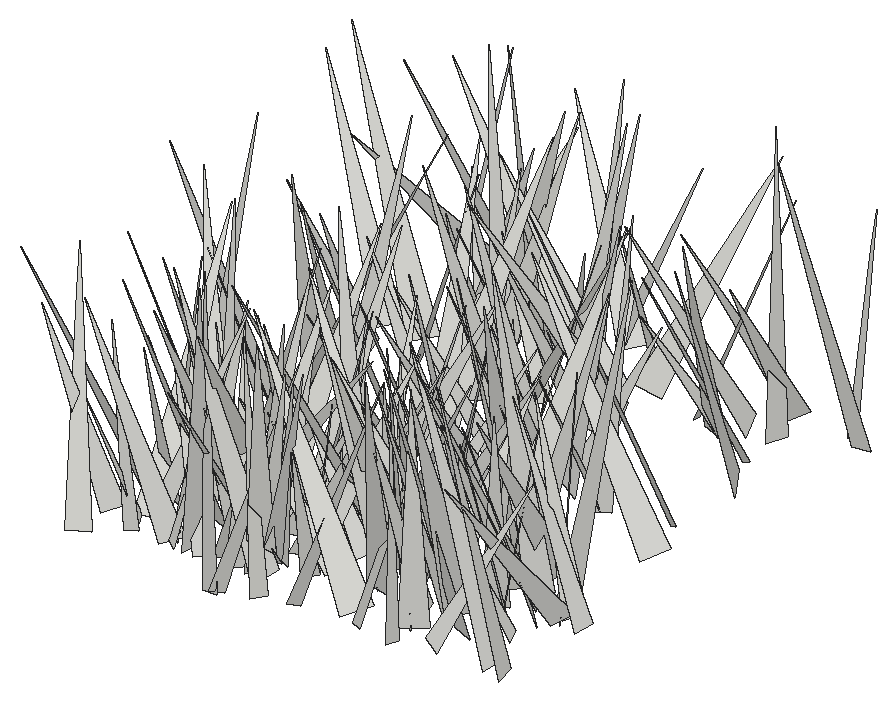
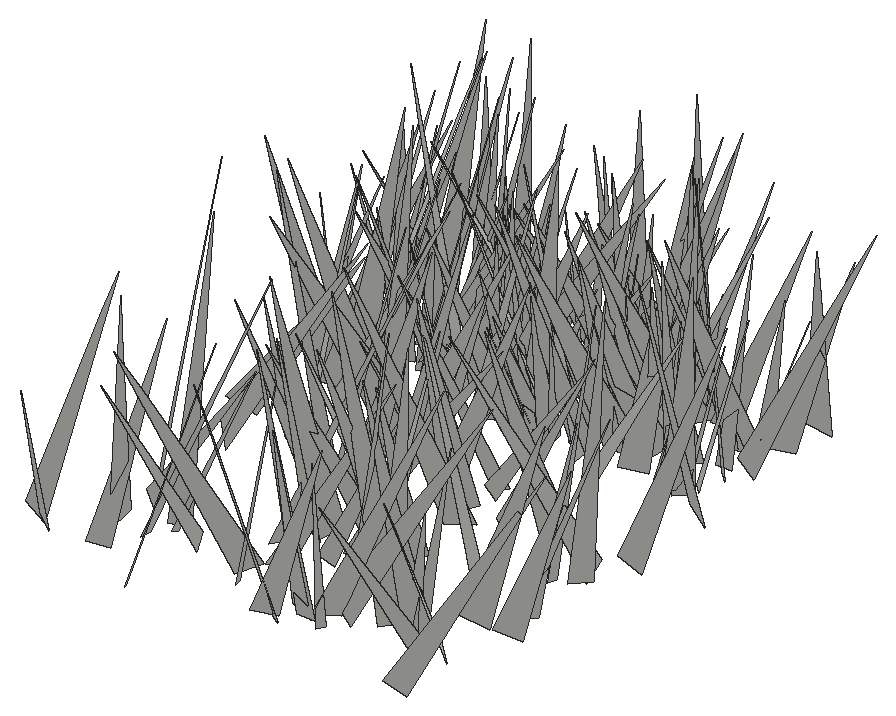
# SketchUp Ruby script. Lengths in inches.
U = 1.inch
M = Sketchup.active_model
def pt(a) = Geom::Point3d.new(a.map { |v| v * U })
def face(e, loops, mat)
  f = e.add_face(loops[0].map { |a| pt(a) })
  loops[1..].each { |l| e.add_face(l.map { |a| pt(a) }).erase! }
  f.material = f.back_material = mat if mat
  f
end
# faces: each face lists its corners as indices into pts; further lists are holes
def faces(e, pts, list, mat = nil) = list.each { |f| face(e, (f[0].is_a?(Array) ? f : [f]).map { |l| l.map { |i| pts[i] } }, mat) }
# xy, xz, yz: faces in a plane at the given z, y or x. An outline is a flat list of corners, or four numbers for a rectangle; further outlines are holes
def ring(l) = l.size == 4 ? [[l[0], l[1]], [l[2], l[1]], [l[2], l[3]], [l[0], l[3]]] : l.each_slice(2).to_a
def flat(e, list, mat, &to3) = list.each { |f| face(e, (f[0].is_a?(Array) ? f : [f]).map { |l| ring(l).map { |u, v| to3.(u, v) } }, mat) }
def xy(e, z, list, mat = nil) = flat(e, list, mat) { |x, y| [x, y, z] }
def xz(e, y, list, mat = nil) = flat(e, list, mat) { |x, z| [x, y, z] }
def yz(e, x, list, mat = nil) = flat(e, list, mat) { |y, z| [x, y, z] }
def lines(e, pts, list) = list.each { |a, b| e.add_line(pt(pts[a]), pt(pts[b])) }
# prism: a flat outline (further loops are holes) pulled along v
def prism(e, loops, v, mat = nil)
  f = face(e, loops, mat); d = Geom::Vector3d.new(v.map { |x| x * U })
  f.pushpull(f.normal.samedirection?(d) ? d.length : -d.length)
end
def box(e, o, s, mat = nil) = prism(e, [[o, [o[0] + s[0], o[1], o[2]], [o[0] + s[0], o[1] + s[1], o[2]], [o[0], o[1] + s[1], o[2]]]], [0, 0, s[2]], mat)
def at(x, y, z, deg = 0) = Geom::Transformation.translation(pt([x, y, z])) * Geom::Transformation.rotation(ORIGIN, Z_AXIS, deg.degrees)
def axes(o, x, y, z) = Geom::Transformation.new([*x, 0, *y, 0, *z, 0, *pt(o).to_a, 1])
def part(name) = M.definitions.add(name)
# library, detail: a bought-in or finely detailed component or shape, given as its bounding box
def library(name, o, s) = part(name).tap { |d| box(d.entities, o, s) }
def detail(e, o, s) = box(e.add_group.entities, o, s)
def put(e, d, t, mat = nil) = e.add_instance(d, t).tap { |i| i.material = mat if mat }
def group(e, t, mat = nil) = e.add_group.tap { |g| g.transformation = t; g.material = mat if mat }.entities
root = M.entities
c1 = part("fur_instance\#9")
p = [[0.8125,0,1.79],[0.67,-0.02,1.48],[0,-0.11,0],[0,0.11,0]]
faces(c1.entities,p,[[0,1,2,3]])
put(root,c1,axes([460.6875,140.12,-21.86],[7.59105,-2.36712,2.02897],[-2.18853,-7.84946,-0.96967],[-2.22043,-0.35586,7.89221]))
put(root,c1,axes([464.49,140.16,-21.86],[5.8288,-3.89293,1.62458],[-3.86791,-6.0381,-0.59132],[-1.68328,0.3943,6.98428]))
put(root,c1,axes([463.9375,137.01,-21.86],[2.76553,6.92914,2.18566],[6.51494,-3.40021,2.53621],[-3.21647,-0.92942,7.01632]))
put(root,c1,axes([464.78,140.87,-21.66],[-1.76635,-5.02439,0.02248],[-4.81779,1.68692,-1.51928],[-1.42615,0.52421,5.10454]))
put(root,c1,axes([455.63,140.11,-21.66],[-4.26864,3.3889,1.68719],[3.78174,3.93314,1.66776],[0.17248,-2.36607,5.18889]))
put(root,c1,axes([459.45,139.79,-21.86],[-3.27496,5.22829,1.96451],[5.47571,2.5569,2.32348],[-1.10043,-2.83671,5.71505]))
put(root,c1,axes([462.74,142,-21.86],[0.98136,-7.62341,0.77855],[-7.49654,-1.11781,-1.49599],[-1.58884,0.56543,7.53933]))
put(root,c1,axes([470.25,142.0625,-21.86],[0.34985,-8.1007,0.677],[-7.9597,-0.20383,1.67442],[1.6501,0.73429,7.93347]))
put(root,c1,axes([465.12,139.72,-21.86],[-8.06314,0.9505,0.88883],[1.02226,8.07835,0.63476],[0.80526,-0.7379,8.09412]))
put(root,c1,axes([479.77,139.47,-21.86],[-7.02647,-2.17808,1.10616],[-2.29777,7.03636,-0.74079],[0.82938,1.04138,7.31892]))
put(root,c1,axes([456.98,140.48,-21.86],[-3.14416,-1.79317,0.28571],[-1.75542,3.14785,0.43854],[0.46429,-0.24163,3.59289]))
put(root,c1,axes([455.63,137.48,-21.66],[-1.06159,6.87885,0.56166],[6.76624,0.92524,1.45707],[-1.36093,-0.76575,6.80607]))
put(root,c1,axes([474.82,142.48,-21.66],[5.51708,-5.76072,0.82028],[-5.55442,-5.55067,-1.6234],[-1.73412,-0.54876,7.80952]))
put(root,c1,axes([464.41,136.92,-21.66],[5.42,0.95377,1.93695],[-0.10115,-5.11614,2.80228],[-2.15667,2.63692,4.73638]))
put(root,c1,axes([473.36,141.42,-21.66],[-6.08575,-1.31512,1.93305],[-0.80976,6.24223,1.69745],[2.19329,-1.34444,5.99037]))
put(root,c1,axes([473.63,140.26,-21.86],[4.24659,-4.94069,2.32668],[-5.22174,-4.53655,-0.10277],[-1.59916,1.69313,6.51409]))
put(root,c1,axes([466.03,138.0625,-21.86],[-6.21207,0.31771,0.7174],[0.09871,5.99609,-1.80072],[0.77837,1.77522,5.95384]))
put(root,c1,axes([473.68,138.58,-21.86],[-5.20455,-0.25594,1.25726],[-0.61037,5.11409,-1.48563],[1.12857,1.58561,4.99457]))
put(root,c1,axes([475.7,141.32,-21.86],[-3.27464,-6.78559,1.40651],[-6.92909,3.22889,-0.5548],[0.10135,1.50857,7.51397]))
put(root,c1,axes([466.7,141.1,-21.86],[2.8154,-3.04723,0.70248],[-2.99803,-2.89898,-0.55973],[-0.88933,0.126,4.11081]))
put(root,c1,axes([478.75,139.99,-21.86],[-8.26176,0.40654,0.83522],[0.41692,8.30295,0.08258],[0.83009,-0.12394,8.27135]))
put(root,c1,axes([464.52,140.88,-21.86],[6.13982,-1.63324,0.91897],[-1.58888,-6.20592,-0.4139],[-0.99371,-0.16841,6.33984]))
put(root,c1,axes([470.73,139.58,-21.66],[-4.85114,5.94494,0.47809],[5.69058,4.42924,2.66526],[-1.78556,-2.03568,7.19529]))
put(root,c1,axes([459.375,140.12,-21.86],[2.36922,2.94645,1.17355],[3.15581,-2.33594,-0.5062],[-0.31572,-1.23846,3.7468]))
put(root,c1,axes([459.64,139.46,-21.86],[2.29816,3.3477,0.63042],[3.39972,-2.30202,-0.16916],[-0.21536,-0.61617,4.05709]))
put(root,c1,axes([464.46,141.57,-21.86],[-0.76172,-5.93829,1.58025],[-5.83151,1.20063,1.7008],[1.93753,1.27903,5.74028]))
put(root,c1,axes([464.05,140.9375,-21.86],[0.25447,-5.59234,1.88155],[-5.79418,0.11887,1.13692],[1.11444,1.89496,5.48146]))
put(root,c1,axes([464.12,141,-21.66],[1.30343,6.50873,4.51627],[7.0846,-3.00591,2.28737],[-3.54523,-3.61388,6.23141]))
put(root,c1,axes([457.35,139.32,-21.86],[0.45308,4.94253,1.25959],[4.74966,-0.86975,1.70432],[-1.859,-1.01755,4.66145]))
put(root,c1,axes([473.06,140.45,-21.86],[3.81307,5.29138,3.34018],[5.75803,-4.49829,0.55278],[-2.44962,-2.33704,6.49867]))
put(root,c1,axes([460.32,142.4,-21.86],[-3.1759,-6.57357,0.78945],[-6.61199,3.10387,-0.75436],[-0.34161,1.03711,7.26148]))
put(root,c1,axes([461.49,139.54,-21.86],[-1.35626,4.67986,0.4324],[4.48876,1.15652,1.56235],[-1.3925,-0.82998,4.61514]))
put(root,c1,axes([474.27,142.13,-21.86],[-5.80555,-2.80529,1.19859],[-2.69051,5.92298,0.83076],[1.43785,-0.24369,6.39405]))
put(root,c1,axes([475.28,139.49,-21.86],[2.06268,4.77096,0.10661],[4.57909,-1.94603,-1.50762],[1.34363,-0.69206,4.97431]))
put(root,c1,axes([455.95,142.52,-21.66],[-2.71774,-6.73125,0.47193],[-6.54696,2.5072,-1.9416],[-1.63394,1.15011,6.99472]))
put(root,c1,axes([464.32,141.84,-21.86],[-3.33376,-1.76985,1.3611],[-1.54667,3.5947,0.88593],[1.61021,-0.21143,3.66899]))
put(root,c1,axes([468.02,138.23,-21.66],[5.42222,1.22065,1.50489],[0.3801,-5.05507,2.73075],[-1.90005,2.47215,4.84081]))
put(root,c1,axes([463.65,139.87,-21.86],[0.20171,6.63601,2.13173],[6.14884,-1.17367,3.07178],[-3.28217,-1.79094,5.8857]))
put(root,c1,axes([457.02,142.83,-21.86],[-0.80762,-5.18,0.70533],[-5.16495,0.90095,0.70267],[0.80822,0.5814,5.19528]))
put(root,c1,axes([477.77,142.53,-21.86],[-4.15133,-1.53142,0.10873],[-1.49707,4.10736,0.69206],[0.34034,-0.61232,4.37033]))
put(root,c1,axes([466.35,141.6,-21.86],[3.95435,2.54343,1.52337],[2.80761,-4.0284,-0.56212],[-0.95239,-1.31514,4.66797]))
put(root,c1,axes([460.26,145.63,-21.86],[7.18044,-3.7228,0.21814],[-3.29243,-6.55088,-3.42221],[-1.75122,-2.94828,7.32847]))
put(root,c1,axes([467.46,142.03,-21.66],[-3.75948,2.94392,0.27379],[2.73653,3.29698,2.12525],[-1.1194,-1.82718,4.27594]))
put(root,c1,axes([461.97,141.26,-21.66],[0.15011,3.96157,1.30257],[3.86973,0.35348,-1.52101],[1.55431,-1.26265,3.66102]))
put(root,c1,axes([478.59,145.29,-21.86],[3.78174,-4.82109,0.17581],[-4.12071,-3.34423,-3.06777],[-2.50869,-1.77444,5.30408]))
put(root,c1,axes([474.12,144.14,-21.66],[-5.52668,-3.91053,1.22579],[-3.5737,5.60606,1.77193],[2.00587,-0.78663,6.53427]))
put(root,c1,axes([463.19,141.96,-21.86],[5.93404,-1.49093,1.99542],[-1.59561,-6.23409,0.08712],[-1.91274,0.57506,6.11785]))
put(root,c1,axes([470.54,144.52,-21.66],[0.16634,-6.6201,0.01552],[-6.42128,-0.15757,1.61124],[1.61035,0.05552,6.42319]))
put(root,c1,axes([474.13,143.64,-21.66],[-7.00038,0.48524,0.02911],[0.47648,6.76613,1.79834],[-0.09628,-1.796,6.78283]))
put(root,c1,axes([477.43,144.62,-21.86],[-4.26482,-5.03014,0.77761],[-4.82923,4.31941,1.45497],[1.60794,-0.36894,6.43227]))
put(root,c1,axes([457.48,141.1,-21.86],[2.30365,5.6713,0.71156],[5.64313,-2.13475,-1.25489],[0.90837,-1.12069,5.9913]))
put(root,c1,axes([475.93,144.27,-21.86],[-3.75985,-4.2409,1.14983],[-3.97997,3.92819,1.47409],[1.86202,-0.16705,5.47255]))
put(root,c1,axes([474.09,143.25,-21.86],[-5.02334,-0.16728,0.55191],[-0.071,4.98153,0.86367],[0.57231,-0.85028,4.95137]))
put(root,c1,axes([461.45,142.83,-21.86],[-5.59942,-5.49473,0.70955],[-5.42162,5.22657,-2.3104],[-1.14084,2.13071,7.49717]))
put(root,c1,axes([471.55,138.53,-21.66],[5.15692,6.28398,0.1894],[5.87834,-4.90651,2.73667],[-2.22922,1.59869,7.6546]))
put(root,c1,axes([470.04,142.79,-21.86],[-6.68615,-0.01766,0.93467],[0.01232,6.74773,0.2156],[0.93476,-0.21523,6.6827]))
put(root,c1,axes([463.9,141.42,-21.66],[1.76698,3.75792,1.11012],[3.4505,-2.06932,1.51278],[-1.85698,-0.26926,3.86726]))
put(root,c1,axes([456.93,146.11,-21.86],[-1.50636,-7.45489,0.25307],[-6.77182,1.47502,3.14252],[3.12761,-0.39686,6.92598]))
put(root,c1,axes([476.27,146.09,-21.86],[-5.99255,-5.60768,0.41861],[-5.37957,5.89507,1.95969],[1.63755,-1.155,7.96972]))
put(root,c1,axes([456.32,143.79,-21.66],[5.45903,4.38742,2.52703],[5.0114,-5.21201,-1.77686],[-0.72192,-3.00365,6.77446]))
put(root,c1,axes([468.18,145.86,-21.86],[6.61822,-2.56323,1.80089],[-1.74555,-6.51281,-2.85492],[-2.60123,-2.15113,6.49773]))
put(root,c1,axes([473.9,144.41,-21.86],[-0.45629,-4.37673,0.42276],[-4.25435,0.54685,1.06962],[1.11127,0.29645,4.26847]))
put(root,c1,axes([469.76,144.03,-21.66],[-3.41379,-7.32141,0.63154],[-6.65452,2.7845,-3.69049],[-3.11756,2.07349,7.18591]))
put(root,c1,axes([464.84,143.125,-21.86],[-3.17,-4.98135,1.74667],[-5.27871,2.99065,-1.05117],[-0.00204,2.03858,5.81015]))
put(root,c1,axes([464.37,144.34,-21.86],[-2.39227,-3.29447,0.41561],[-3.24315,2.42809,0.57931],[0.71291,-0.00928,4.03]))
put(root,c1,axes([464.96,142.47,-21.86],[4.25693,-2.37845,0.80532],[-2.50825,-3.95225,1.586],[0.11926,1.77474,4.61119]))
put(root,c1,axes([475.33,144.33,-21.86],[3.25628,-4.96201,1.27437],[-5.08219,-3.31911,0.06246],[-0.64574,1.10043,5.93473]))
put(root,c1,axes([462.47,139.63,-21.66],[-6.96158,0.42843,3.50828],[-1.43896,6.73486,-3.67782],[3.22816,3.92599,5.92628]))
put(root,c1,axes([461.75,142.05,-21.86],[-4.60941,2.24833,0.68921],[2.12734,4.63308,-0.88638],[1.00221,0.50623,5.05134]))
put(root,c1,axes([470.87,144.93,-21.86],[7.66511,2.45698,1.17946],[2.70747,-7.26796,-2.45522],[-0.3122,-2.70587,7.66567]))
put(root,c1,axes([469.67,145.18,-21.86],[-4.01189,-2.17426,1.82805],[-1.57492,4.33524,1.69992],[2.36407,-0.80168,4.23473]))
put(root,c1,axes([468.37,145.51,-21.66],[3.73723,-3.51523,0.8829],[-3.22394,-3.80362,-1.49732],[-1.65607,-0.52811,4.90732]))
put(root,c1,axes([466.13,141.95,-21.66],[1.18506,6.07091,0.5983],[5.8889,-0.9794,-1.72625],[1.5921,-0.89616,5.93973]))
put(root,c1,axes([463.65,145.1875,-21.86],[3.35042,-5.0359,1.55374],[-4.92978,-3.64566,-1.18576],[-1.86322,0.59037,5.93123]))
put(root,c1,axes([468.98,144.34,-21.86],[0.54293,-5.17192,1.62827],[-5.42158,-0.49338,0.24063],[0.08095,1.64396,5.19477]))
put(root,c1,axes([462.79,141.52,-21.86],[0.90222,6.95991,0.72818],[6.98982,-0.93156,0.24337],[-0.33621,-0.69025,7.01392]))
put(root,c1,axes([458.55,143.3,-21.86],[-0.43128,5.47544,2.09207],[5.72554,0.84273,-1.02531],[1.25517,-1.9628,5.39585]))
put(root,c1,axes([456.76,145.11,-21.86],[-3.11694,-3.18155,0.61605],[-3.14817,3.17551,0.47138],[0.76862,0.10457,4.42892]))
put(root,c1,axes([460.12,143.85,-21.66],[4.62991,-4.98565,0.093],[-4.3743,-3.99984,3.34189],[2.39393,2.33366,5.92659]))
put(root,c1,axes([475.04,146.28,-21.86],[2.63198,-5.20128,0.6124],[-4.94839,-2.69423,-1.6156],[-1.71515,-0.20845,5.60093]))
put(root,c1,axes([457.3,140.89,-21.86],[-3.2389,7.2108,0.31573],[7.08918,3.2432,-1.34571],[1.35602,0.26802,7.78942]))
put(root,c1,axes([467.45,144.32,-21.86],[-3.7614,2.09395,0.36046],[2.10674,3.58022,1.1859],[-0.27609,-1.20834,4.13841]))
put(root,c1,axes([463.6,143.41,-21.66],[3.57113,-2.0967,0.79041],[-2.23153,-3.1932,1.61171],[0.20288,1.78359,3.81464]))
put(root,c1,axes([457.93,144.27,-21.86],[-2.9488,-2.48385,0.84804],[-2.61567,2.88641,-0.64107],[0.2167,1.04076,3.80183]))
put(root,c1,axes([477.28,142.09,-21.86],[4.44395,3.96646,1.43413],[3.47391,-4.62357,2.02305],[-2.39195,0.65422,5.60257]))
put(root,c1,axes([459.07,145.42,-21.86],[-3.51503,-1.89548,0.64915],[-1.82323,3.56963,0.55065],[0.83071,-0.18586,3.95538]))
put(root,c1,axes([461.625,143.05,-21.86],[-0.94911,6.39885,1.08787],[6.32075,1.1611,-1.31509],[1.4754,-0.85797,6.33377]))
put(root,c1,axes([476.15,148.39,-21.66],[4.64507,-4.79979,0.2726],[-4.36308,-4.36804,-2.56373],[-2.01887,-1.6035,6.16782]))
put(root,c1,axes([465.91,146.23,-21.66],[5.21952,0.68023,0.61562],[0.83808,-4.98198,-1.60081],[-0.37326,-1.674,5.01433]))
put(root,c1,axes([465.2,145.33,-21.86],[5.8637,3.4963,0.04079],[3.31459,-5.53283,-2.23832],[1.11324,-1.94227,6.44958]))
put(root,c1,axes([469.15,144.28,-21.86],[-5.54363,5.04114,0.10568],[4.92423,5.3789,1.72499],[-1.08457,-1.34553,7.29173]))
put(root,c1,axes([462.96,146.27,-21.86],[6.83601,2.20523,1.02382],[2.40175,-6.59991,-1.82073],[-0.37792,-2.05437,6.94831]))
put(root,c1,axes([458.59,145.45,-21.86],[-2.19445,-3.56039,1.55722],[-3.85398,2.22319,-0.34801],[0.4981,1.5159,4.16783]))
put(root,c1,axes([479.89,145.26,-21.86],[-5.92651,0.06077,0.05927],[0.05827,5.92175,-0.24529],[0.06173,0.24468,5.92174]))
put(root,c1,axes([462.11,144.73,-21.86],[-0.06431,5.36711,1.48252],[5.54585,0.19413,-0.46222],[0.49719,-1.47116,5.34755]))
put(root,c1,axes([469.03,145.35,-21.86],[-4.7956,1.01448,1.55419],[0.95492,5.04106,-0.34401],[1.59148,0.0322,4.88965]))
put(root,c1,axes([478.83,145.875,-21.86],[-5.29366,2.0126,1.17564],[2.12712,5.36423,0.39489],[0.95291,-0.79376,5.64955]))
put(root,c1,axes([466.85,144.79,-21.66],[-1.50956,7.97784,1.83345],[8.07703,1.14872,1.65178],[-1.3301,-2.07864,7.94961]))
put(root,c1,axes([467.5625,145.76,-21.86],[5.25696,-1.00652,0.21452],[-1.02902,-5.15697,1.02054],[-0.01477,1.04274,5.25426]))
put(root,c1,axes([458.59,144.67,-21.66],[1.63726,6.8228,1.57078],[6.72877,-1.9791,1.58281],[-1.9343,-1.10957,6.83563]))
put(root,c1,axes([472.35,144.39,-21.66],[-2.22642,5.28944,0.76409],[4.89566,2.35054,-2.00661],[2.14349,0.12554,5.37668]))
put(root,c1,axes([473.4375,146.5,-21.86],[1.95636,4.4496,1.57567],[4.70552,-1.97342,-0.26957],[-0.3738,-1.55425,4.8532]))
put(root,c1,axes([464.87,145.82,-21.86],[-3.84179,0.25674,0.88435],[-0.00822,3.78425,-1.13434],[0.92083,1.10494,3.67947]))
put(root,c1,axes([476.19,146.52,-21.66],[-0.9931,7.68396,2.84346],[8.04191,0.36629,1.81887],[-1.56723,-2.98953,7.53135]))
put(root,c1,axes([478.72,144.9,-21.86],[3.82585,4.29132,1.89582],[3.55577,-4.24822,2.44044],[-3.06039,0.42878,5.20545]))
put(root,c1,axes([466.42,145.18,-21.86],[-4.08665,1.67614,0.95166],[1.15635,3.91687,-1.93308],[1.54207,1.50482,3.97156]))
put(root,c1,axes([466.82,145.23,-21.86],[2.09645,3.63188,0.13416],[3.39461,-2.01213,1.42535],[-1.29816,0.60366,3.94386]))
put(root,c1,axes([465.09,146.02,-21.86],[-4.76791,1.69378,1.39092],[1.4281,4.92716,-1.10462],[1.66255,0.62512,4.93778]))
put(root,c1,axes([461.92,144.35,-21.66],[-4.61251,5.93847,1.25396],[5.3205,4.71401,-2.75381],[2.92064,0.79104,6.99694]))
put(root,c1,axes([457.47,145.8,-21.86],[-5.44191,5.3364,0.6963],[5.36336,5.45938,0.07682],[0.44311,-0.54257,7.6214]))
put(root,c1,axes([467.48,144.79,-21.86],[-4.827,3.94667,0.05385],[3.76525,4.62978,-1.80751],[1.18405,1.36675,5.96733]))
put(root,c1,axes([461.29,147.28,-21.66],[-4.82792,-3.85999,0.34861],[-3.62589,4.30173,-2.58417],[-1.36894,2.21934,5.6152]))
put(root,c1,axes([463.14,145.64,-21.86],[0.33819,7.69063,1.05021],[7.70297,-0.20312,-0.99305],[0.95553,-1.08446,7.63374]))
put(root,c1,axes([468.7,148.42,-21.66],[4.45492,4.83666,0.95124],[4.56601,-3.56591,-3.25273],[1.85733,-2.83468,5.71483]))
put(root,c1,axes([470.35,146.75,-21.86],[3.87453,3.49507,1.24049],[3.40824,-4.0629,0.80191],[-1.46226,-0.20898,5.15601]))
put(root,c1,axes([474.04,147.8,-21.66],[-6.46812,-3.13785,1.21731],[-3.3431,6.29489,-1.53709],[0.38946,1.92167,7.02282]))
put(root,c1,axes([466.18,151.38,-21.66],[-2.99336,-6.46525,0.18966],[-6.30073,2.9619,1.52434],[1.46161,-0.47255,6.9596]))
put(root,c1,axes([470.27,151.83,-21.66],[7.22069,-3.00234,1.05262],[-2.62839,-7.10035,-2.22196],[-1.79266,-1.6827,7.49769]))
put(root,c1,axes([478.01,146.29,-21.86],[7.23662,0.86237,3.59764],[-0.54989,-7.56504,2.91946],[-3.65846,2.84288,6.67751]))
put(root,c1,axes([469.38,151.91,-21.66],[1.60402,-6.13136,0.73735],[-5.58582,-1.76536,-2.52831],[-2.63361,0.00991,5.81155]))
put(root,c1,axes([474.78,149.99,-21.66],[-4.9499,-5.12629,0.49866],[-4.98162,4.58947,-2.26921],[-1.30806,1.92014,6.75508]))
put(root,c1,axes([474.51,147.63,-21.66],[6.67924,-1.26552,2.75336],[-2.18749,-6.62541,2.26131],[-2.097,2.88046,6.41095]))
put(root,c1,axes([454.89,147.49,-21.66],[3.59561,7.30217,1.1805],[7.09033,-3.77639,1.76345],[-2.10771,-0.24675,7.94609]))
put(root,c1,axes([463.92,151.84,-21.66],[-1.49578,-4.28811,0.26565],[-3.87905,1.22698,-2.03551],[-1.84701,0.89578,4.0598]))
put(root,c1,axes([472.74,155.14,-21.66],[-3.72735,-5.65721,0.3773],[-4.71825,3.34531,3.54775],[3.14396,-1.68653,5.77153]))
put(root,c1,axes([467.91,151.07,-21.66],[-2.85535,-4.62994,1.75531],[-4.89429,2.33192,-1.81068],[-0.75056,2.40755,5.12941]))
put(root,c1,axes([471.26,154.04,-21.66],[-5.10979,-2.8974,1.28802],[-2.4355,5.15064,1.92434],[2.03034,-1.11347,5.54994]))
put(root,c1,axes([463.72,151.23,-21.66],[1.55014,5.60518,1.20615],[5.3228,-0.94254,-2.46072],[2.13086,-1.72318,5.26933]))
put(root,c1,axes([466.02,152.5,-21.66],[-3.70212,4.89762,1.86065],[5.19102,3.12087,2.11373],[-0.70854,-2.72541,5.76407]))
put(root,c1,axes([454.44,153.14,-21.66],[-0.79345,-6.87819,1.77521],[-6.83318,0.25089,-2.08208],[-1.94125,1.92821,6.60333]))
put(root,c1,axes([472.59,148.58,-21.66],[-6.00676,5.62271,0.83771],[4.81686,5.68135,-3.59416],[3.01902,2.12255,7.40122]))
put(root,c1,axes([468.35,154.01,-21.66],[-2.5232,4.5633,1.53247],[4.25008,1.29942,3.12842],[-2.26029,-2.65076,4.17172]))
put(root,c1,axes([466.23,152.69,-21.66],[1.55212,3.88569,0.28277],[3.69063,-1.36892,-1.44671],[1.24813,-0.78428,3.92616]))
put(root,c1,axes([478.31,152.58,-21.66],[-3.77529,6.85051,0.02559],[5.94676,3.26269,3.89536],[-3.40091,-1.89957,6.78296]))
put(root,c1,axes([461.41,154.18,-21.66],[-3.32714,-4.87132,0.7615],[-4.7527,2.92423,-2.05917],[-1.31203,1.7603,5.52806]))
put(root,c1,axes([455.2,155.94,-21.66],[6.33398,-2.31725,1.64534],[-1.9481,-6.46653,-1.60778],[-2.06922,-1.00519,6.55011]))
put(root,c1,axes([456.36,156.625,-21.66],[6.05103,1.03829,2.78411],[2.19851,-5.8136,-2.61017],[-1.99898,-3.2509,5.55698]))
put(root,c1,axes([466.42,156.51,-21.66],[-7.9399,0.37328,2.34081],[0.92834,8.01881,1.87016],[2.18103,-2.05426,7.72553]))
put(root,c1,axes([471.04,155.01,-21.66],[-2.12698,-6.60371,3.80122],[-7.1046,3.14508,1.48842],[2.75369,3.0136,6.77625]))
put(root,c1,axes([477.26,155.29,-21.66],[-5.76145,-5.93812,0.42997],[-5.44241,5.01036,-3.73055],[-2.41379,2.87671,7.38502]))
put(root,c1,axes([468.77,155.92,-21.66],[-0.03383,-6.90938,2.82252],[-7.12958,-0.80509,-2.05628],[-2.20801,2.70547,6.5964]))
put(root,c1,axes([459.17,152.87,-21.66],[-6.96616,2.88196,1.8212],[2.05018,6.85162,-3.00033],[2.72382,2.21349,6.91601]))
put(root,c1,axes([463.91,153.97,-21.66],[-5.45003,5.37343,0.92209],[5.18096,5.51046,-1.48977],[1.69756,0.43353,7.50714]))
put(root,c1,axes([470.51,156.74,-21.66],[0.36945,4.73641,1.83647],[4.53767,0.52011,-2.25427],[2.28381,-1.79961,4.18191]))
put(root,c1,axes([455.34,154.71,-21.66],[7.33228,1.89466,0.16833],[1.78282,-7.07911,2.02191],[-0.66303,1.91751,7.29821]))
put(root,c1,axes([477.05,160.35,-21.66],[-6.01376,-4.74049,2.00405],[-3.98095,6.23797,2.80955],[3.26197,-1.12665,7.12348]))
put(root,c1,axes([473.85,154.3125,-21.66],[2.20032,6.76237,0.49836],[6.15454,-2.21163,2.83722],[-2.84601,0.44546,6.52083]))
put(root,c1,axes([463.13,155.08,-21.66],[-0.97355,8.05143,1.14446],[7.84551,1.23329,-2.00251],[2.14086,-0.85824,7.85896]))
put(root,c1,axes([468.01,155.65,-21.66],[4.5765,3.32185,0.66717],[3.07667,-4.544,1.52],[-1.41913,0.86116,5.4469]))
put(root,c1,axes([468.84,161.9,-21.66],[-7.67561,-3.02253,0.64542],[-2.50236,7.09168,3.4516],[1.81396,-3.00659,7.49247]))
put(root,c1,axes([454.91,160.01,-21.66],[-4.32761,-0.50237,2.11035],[0.41917,4.42689,1.9134],[2.12844,-1.89326,3.91401]))
put(root,c1,axes([455.43,159.9,-21.66],[-5.22696,-1.19875,0.73288],[-0.94186,5.08442,1.59898],[1.04259,-1.41663,5.11873]))
put(root,c1,axes([458.29,159.56,-21.66],[6.75177,1.95337,0.7466],[2.07523,-6.56983,-1.57805],[-0.25785,-1.72661,6.84922]))
put(root,c1,axes([462.6,162.56,-21.66],[-3.43989,-5.36661,0.1848],[-4.97328,3.26677,2.29397],[2.02515,-1.09328,5.94736]))
put(root,c1,axes([465.14,158.75,-21.66],[5.97099,-0.01983,0.33196],[-0.11666,-5.7151,1.75709],[-0.31141,1.76085,5.70664]))
put(root,c1,axes([473.41,163.39,-21.66],[-0.94018,-7.50089,0.47804],[-7.29693,1.02641,1.75419],[1.80188,0.24278,7.35324]))
put(root,c1,axes([465.87,161.72,-21.66],[0.12283,-4.44104,1.09952],[-4.1986,-0.54638,-1.73783],[-1.81756,0.96203,4.08875]))
put(root,c1,axes([462.5,159.1,-21.66],[4.91626,-1.03874,2.91243],[-2.03601,-5.20453,1.58061],[-2.3272,2.35896,4.76972]))
put(root,c1,axes([467.35,159.59,-21.66],[-6.57541,3.25527,2.97746],[2.73361,7.20101,-1.83599],[3.46258,0.49673,7.10365]))
put(root,c1,axes([465.07,160.79,-21.66],[-1.27036,4.00789,0.19304],[3.62684,1.0603,1.85365],[-1.71652,-0.72583,3.77372]))
put(root,c1,axes([476.07,162.25,-21.66],[-2.89235,-4.23355,0.19447],[-3.82387,2.50545,-2.32964],[-1.82723,1.45817,4.56743]))
put(root,c1,axes([473.21,163.93,-21.66],[-4.08154,-1.42978,0.42723],[-1.12455,3.76494,1.85644],[0.98091,-1.633,3.906]))
put(root,c1,axes([474.08,165.07,-21.66],[-6.53247,-2.60599,0.49941],[-2.30056,6.22381,2.3844],[1.32211,-2.04617,6.61657]))
put(root,c1,axes([468.03,160.125,-21.66],[2.36714,6.37429,1.14743],[6.22522,-2.57637,1.46983],[-1.78738,-0.5313,6.63886]))
put(root,c1,axes([458.12,164.37,-21.66],[4.10212,-1.60455,0.85508],[-1.23063,-4.00368,-1.60913],[-1.3384,-1.23658,4.10033]))
put(root,c1,axes([467.38,163.48,-21.66],[-6.03456,2.61232,0.13904],[2.52964,5.73798,1.98392],[-0.66667,-1.87372,6.2693]))
put(root,c1,axes([461.77,160.98,-21.66],[6.32729,-2.1008,2.73388],[-3.01636,-6.1404,2.26257],[-1.67006,3.13117,6.27127]))
put(root,c1,axes([462.29,161.26,-21.66],[0.0482,8.00911,1.76337],[7.92916,-0.49572,2.03478],[-2.09374,-1.69294,7.74648]))
put(root,c1,axes([454.68,162.07,-21.66],[-3.24359,5.98487,0.42852],[5.75195,2.96279,2.1587],[-1.708,-1.38792,6.45597]))
put(root,c1,axes([456.8,162,-21.66],[-3.17251,7.14398,0.8627],[6.87917,2.73438,2.65436],[-2.11131,-1.82544,7.35225]))
put(root,c1,axes([459.48,164.47,-21.66],[3.88235,-7.18309,1.19208],[-7.15051,-3.50623,2.16032],[1.37403,2.04942,7.87416]))
put(root,c1,axes([463.2,162.92,-21.66],[-7.60319,-2.30719,2.08818],[-2.71089,7.61771,-1.45385],[1.52798,2.03457,7.8114]))
put(root,c1,axes([458.13,164.5,-21.66],[3.9818,-4.86666,0.84742],[-4.90357,-3.76221,1.43455],[0.59785,1.55519,6.12218]))
put(root,c1,axes([475.25,167.21,-21.66],[4.02503,-3.95124,0.17731],[-3.62061,-3.78264,-2.10414],[-1.59215,-1.38705,5.23314]))
put(root,c1,axes([467.77,166.03,-21.66],[-3.99319,-2.60087,1.40659],[-2.16034,4.18012,1.59628],[2.0189,-0.6713,4.49021]))
put(root,c1,axes([459.36,163.23,-21.66],[-0.27528,4.26527,0.41219],[4.05575,0.12601,1.40472],[-1.38323,-0.47937,4.03672]))
put(root,c1,axes([462.17,165.1875,-21.66],[-3.051,-7.21191,1.32168],[-6.61753,2.09219,-3.8598],[-3.15701,2.58422,6.81338]))
put(root,c1,axes([462.61,165.83,-21.66],[-6.95314,3.37085,0.59923],[3.40426,6.66259,2.02209],[-0.36434,-2.07731,7.45788]))
put(root,c1,axes([462.06,166.95,-21.66],[-0.71595,-3.844,0.50308],[-3.36107,0.87042,1.86752],[1.93201,0.08975,3.4353]))
put(root,c1,axes([455.6875,169.34,-21.66],[3.04305,-5.48081,0.27728],[-4.42438,-2.6378,-3.58374],[-3.24669,-1.54241,5.14356]))
put(root,c1,axes([479.53,166.62,-21.66],[-2.64388,-6.79077,2.11498],[-6.99476,2.07362,-2.08599],[-1.28885,2.67645,6.98236]))
put(root,c1,axes([471.73,169.58,-21.66],[-4.9139,-3.74374,0.55427],[-3.15126,4.55055,2.79845],[2.0958,-1.9355,5.50733]))
put(root,c1,axes([475.89,164.8,-21.66],[-7.47088,0.3057,1.86762],[-0.12287,7.51123,-1.721],[1.88848,1.69808,7.27638]))
put(root,c1,axes([463.24,166.61,-21.66],[2.35807,6.09522,2.44102],[6.53945,-1.94795,-1.45322],[0.58808,-2.77931,6.37184]))
put(root,c1,axes([471.66,164.05,-21.66],[5.28462,2.45266,0.54887],[2.09175,-5.00051,2.20534],[-1.39334,1.79538,5.39252]))
put(root,c1,axes([468.21,164.65,-21.66],[-2.47927,6.31853,1.78834],[5.49074,3.04318,-3.14001],[3.60191,-0.28983,6.01756]))
put(root,c1,axes([464.15,167.7,-21.66],[4.41432,4.17138,0.78555],[4.1779,-4.06951,-1.86761],[0.75011,-1.88212,5.77916]))
put(root,c1,axes([456.86,165.8,-21.66],[-1.28039,5.01222,0.36244],[4.5705,1.31696,-2.06622],[2.08908,0.19072,4.74262]))
put(root,c1,axes([456.03,165.18,-21.66],[3.80784,5.11048,0.67094],[4.57882,-3.73693,2.47721],[-2.36675,0.99257,5.87197]))
put(root,c1,axes([463.74,166.26,-21.66],[1.51119,6.34193,0.92742],[6.21067,-1.68435,1.39797],[-1.58356,-0.55387,6.36784]))
put(root,c1,axes([465.05,167.47,-21.66],[-4.13597,4.87198,0.25098],[4.78591,3.98836,1.44689],[-0.94567,-1.12348,6.22487]))
put(root,c1,axes([478.6,167.0625,-21.66],[2.37609,4.94692,0.8109],[4.47755,-2.49789,2.11838],[-2.25414,0.25283,5.06264]))
